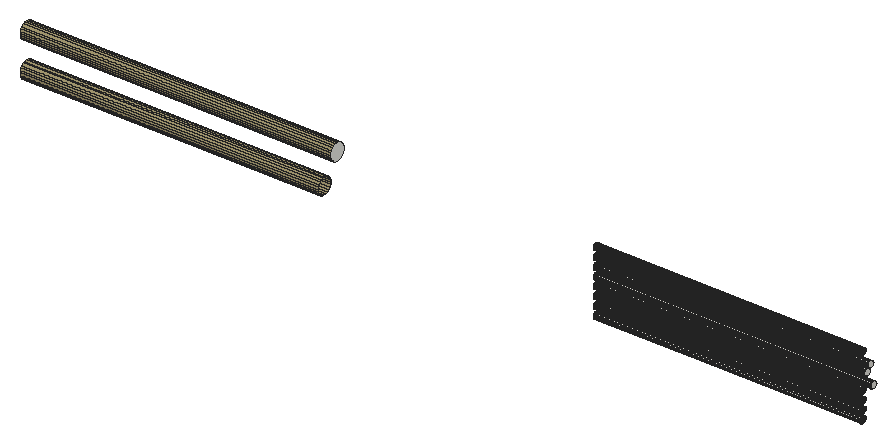
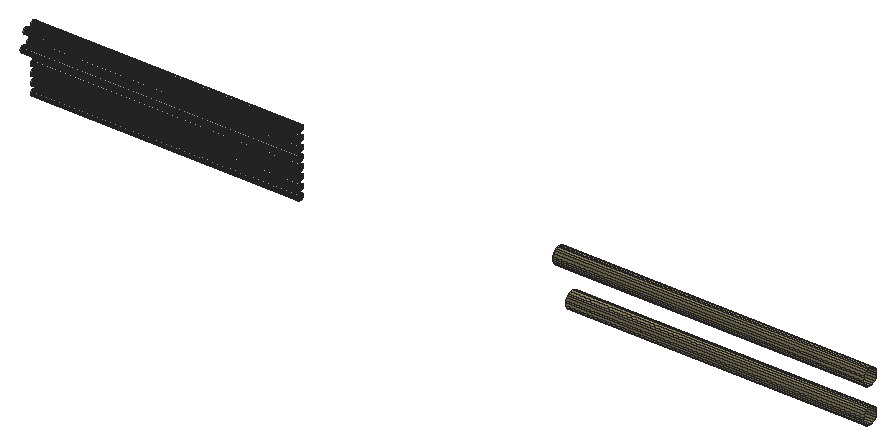
# SketchUp Ruby script. Lengths in inches.
U = 1.inch
M = Sketchup.active_model
def pt(a) = Geom::Point3d.new(a.map { |v| v * U })
def face(e, loops, mat)
  f = e.add_face(loops[0].map { |a| pt(a) })
  loops[1..].each { |l| e.add_face(l.map { |a| pt(a) }).erase! }
  f.material = f.back_material = mat if mat
  f
end
# faces: each face lists its corners as indices into pts; further lists are holes
def faces(e, pts, list, mat = nil) = list.each { |f| face(e, (f[0].is_a?(Array) ? f : [f]).map { |l| l.map { |i| pts[i] } }, mat) }
# xy, xz, yz: faces in a plane at the given z, y or x. An outline is a flat list of corners, or four numbers for a rectangle; further outlines are holes
def ring(l) = l.size == 4 ? [[l[0], l[1]], [l[2], l[1]], [l[2], l[3]], [l[0], l[3]]] : l.each_slice(2).to_a
def flat(e, list, mat, &to3) = list.each { |f| face(e, (f[0].is_a?(Array) ? f : [f]).map { |l| ring(l).map { |u, v| to3.(u, v) } }, mat) }
def xy(e, z, list, mat = nil) = flat(e, list, mat) { |x, y| [x, y, z] }
def xz(e, y, list, mat = nil) = flat(e, list, mat) { |x, z| [x, y, z] }
def yz(e, x, list, mat = nil) = flat(e, list, mat) { |y, z| [x, y, z] }
def lines(e, pts, list) = list.each { |a, b| e.add_line(pt(pts[a]), pt(pts[b])) }
# prism: a flat outline (further loops are holes) pulled along v
def prism(e, loops, v, mat = nil)
  f = face(e, loops, mat); d = Geom::Vector3d.new(v.map { |x| x * U })
  f.pushpull(f.normal.samedirection?(d) ? d.length : -d.length)
end
def box(e, o, s, mat = nil) = prism(e, [[o, [o[0] + s[0], o[1], o[2]], [o[0] + s[0], o[1] + s[1], o[2]], [o[0], o[1] + s[1], o[2]]]], [0, 0, s[2]], mat)
def at(x, y, z, deg = 0) = Geom::Transformation.translation(pt([x, y, z])) * Geom::Transformation.rotation(ORIGIN, Z_AXIS, deg.degrees)
def axes(o, x, y, z) = Geom::Transformation.new([*x, 0, *y, 0, *z, 0, *pt(o).to_a, 1])
def part(name) = M.definitions.add(name)
# library, detail: a bought-in or finely detailed component or shape, given as its bounding box
def library(name, o, s) = part(name).tap { |d| box(d.entities, o, s) }
def detail(e, o, s) = box(e.add_group.entities, o, s)
def put(e, d, t, mat = nil) = e.add_instance(d, t).tap { |i| i.material = mat if mat }
def group(e, t, mat = nil) = e.add_group.tap { |g| g.transformation = t; g.material = mat if mat }.entities
root = M.entities
M.materials.add("[Terrazzo Tile Light]").color = [219, 217, 210]
M.materials.add("[Wood Lumber ButtJoined]").color = [164, 152, 112]
yz(root,389.28,[[249.32,189.85,249.99,189.94,250.6,190.2,251.14,190.6,251.54,191.13,251.8,191.75,251.89,192.42,251.8,193.08,251.54,193.7,251.14,194.23,250.6,194.63,249.99,194.89,249.32,194.98,248.66,194.89,248.04,194.63,247.51,194.23,247.1,193.7,246.85,193.08,246.76,192.42,246.85,191.75,247.1,191.13,247.51,190.6,248.04,190.2,248.66,189.94]])
yz(root,558.48,[[245.69,190.45,245.94,190.48,246.16,190.58,246.36,190.73,246.5,190.92,246.6,191.15,246.63,191.39,246.6,191.63,246.5,191.86,246.36,192.05,246.16,192.2,245.94,192.29,245.69,192.33,245.45,192.29,245.22,192.2,245.03,192.05,244.88,191.86,244.79,191.63,244.75,191.39,244.79,191.15,244.88,190.92,245.03,190.73,245.22,190.58,245.45,190.48]],"[Terrazzo Tile Light]")
yz(root,559.54,[[245.69,193.2,245.94,193.23,246.16,193.33,246.36,193.48,246.5,193.67,246.6,193.9,246.63,194.14,246.6,194.38,246.5,194.61,246.36,194.8,246.16,194.95,245.94,195.04,245.69,195.08,245.45,195.04,245.22,194.95,245.03,194.8,244.88,194.61,244.79,194.38,244.75,194.14,244.79,193.9,244.88,193.67,245.03,193.48,245.22,193.33,245.45,193.23]],"[Terrazzo Tile Light]")
yz(root,560.48,[[245.69,187.7,245.94,187.73,246.16,187.83,246.36,187.98,246.5,188.17,246.6,188.4,246.63,188.64,246.6,188.88,246.5,189.11,246.36,189.3,246.16,189.45,245.94,189.54,245.69,189.58,245.45,189.54,245.22,189.45,245.03,189.3,244.88,189.11,244.79,188.88,244.75,188.64,244.79,188.4,244.88,188.17,245.03,187.98,245.22,187.83,245.45,187.73]],"[Terrazzo Tile Light]")
p = [[473.23,245.22,176.83],[473.23,245.45,176.73],[557.23,245.45,176.73],[557.23,245.22,176.83],[473.23,245.69,176.7],[557.23,245.69,176.7],
  [473.23,245.94,176.73],[557.23,245.94,176.73],[473.23,246.16,176.83],[557.23,246.16,176.83],[473.23,245.03,176.98],[557.23,245.03,176.98],
  [473.23,246.36,176.98],[557.23,246.36,176.98],[473.23,244.88,177.17],[557.23,244.88,177.17],[473.23,246.5,177.17],[557.23,246.5,177.17],
  [473.23,244.79,177.4],[557.23,244.79,177.4],[473.23,246.6,177.4],[557.23,246.6,177.4],[473.23,244.75,177.64],[557.23,244.75,177.64],
  [473.23,246.63,177.64],[557.23,246.63,177.64],[473.23,244.79,177.88],[557.23,244.79,177.88],[473.23,246.6,177.88],[557.23,246.6,177.88],
  [473.23,244.88,178.11],[557.23,244.88,178.11],[473.23,246.5,178.11],[557.23,246.5,178.11],[473.23,245.03,178.3],[557.23,245.03,178.3],
  [473.23,246.36,178.3],[557.23,246.36,178.3],[473.23,245.22,178.45],[557.23,245.22,178.45],[473.23,246.16,178.45],[557.23,246.16,178.45],
  [473.23,245.45,178.54],[557.23,245.45,178.54],[473.23,245.69,178.58],[557.23,245.69,178.58],[473.23,245.94,178.54],[557.23,245.94,178.54],
  [291.78,248.04,179.2],[291.78,248.66,178.94],[385.09,248.66,178.94],[385.09,248.04,179.2],[291.78,249.32,178.85],[385.09,249.32,178.85],
  [291.78,249.99,178.94],[385.09,249.99,178.94],[291.78,250.6,179.2],[385.09,250.6,179.2],[291.78,247.51,179.6],[385.09,247.51,179.6],
  [291.78,251.14,179.6],[385.09,251.14,179.6],[473.23,245.22,179.58],[473.23,245.45,179.48],[557.23,245.45,179.48],[557.23,245.22,179.58],
  [473.23,245.69,179.45],[557.23,245.69,179.45],[473.23,245.94,179.48],[557.23,245.94,179.48],[473.23,246.16,179.58],[557.23,246.16,179.58],
  [473.23,245.03,179.73],[557.23,245.03,179.73],[473.23,246.36,179.73],[557.23,246.36,179.73],[291.78,247.1,180.13],[385.09,247.1,180.13],
  [291.78,251.54,180.13],[385.09,251.54,180.13],[473.23,244.88,179.92],[557.23,244.88,179.92],[473.23,246.5,179.92],[557.23,246.5,179.92],
  [473.23,244.79,180.15],[557.23,244.79,180.15],[473.23,246.6,180.15],[557.23,246.6,180.15],[473.23,244.75,180.39],[557.23,244.75,180.39],
  [473.23,246.63,180.39],[557.23,246.63,180.39],[291.78,246.85,180.75],[385.09,246.85,180.75],[291.78,251.8,180.75],[385.09,251.8,180.75],
  [473.23,244.79,180.63],[557.23,244.79,180.63],[473.23,246.6,180.63],[557.23,246.6,180.63],[473.23,244.88,180.86],[557.23,244.88,180.86],
  [473.23,246.5,180.86],[557.23,246.5,180.86],[291.78,246.76,181.42],[385.09,246.76,181.42],[291.78,251.89,181.42],[385.09,251.89,181.42],
  [473.23,245.03,181.05],[557.23,245.03,181.05],[473.23,246.36,181.05],[557.23,246.36,181.05],[473.23,245.22,181.2],[557.23,245.22,181.2],
  [473.23,246.16,181.2],[557.23,246.16,181.2],[473.23,245.45,181.29],[557.23,245.45,181.29],[473.23,245.94,181.29],[557.23,245.94,181.29],
  [473.23,245.69,181.33],[557.23,245.69,181.33],[291.78,246.85,182.08],[385.09,246.85,182.08],[291.78,251.8,182.08],[385.09,251.8,182.08],
  [291.78,247.1,182.7],[385.09,247.1,182.7],[291.78,251.54,182.7],[385.09,251.54,182.7],[473.23,245.22,182.33],[473.23,245.45,182.23],
  [557.23,245.45,182.23],[557.23,245.22,182.33],[473.23,245.69,182.2],[557.23,245.69,182.2],[473.23,245.94,182.23],[557.23,245.94,182.23],
  [473.23,246.16,182.33],[557.23,246.16,182.33],[473.23,245.03,182.48],[557.23,245.03,182.48],[473.23,246.36,182.48],[557.23,246.36,182.48],
  [473.23,244.88,182.67],[557.23,244.88,182.67],[473.23,246.5,182.67],[557.23,246.5,182.67],[473.23,244.79,182.9],[557.23,244.79,182.9],
  [473.23,246.6,182.9],[557.23,246.6,182.9],[291.78,247.51,183.23],[385.09,247.51,183.23],[291.78,251.14,183.23],[385.09,251.14,183.23],
  [473.23,244.75,183.14],[557.23,244.75,183.14],[473.23,246.63,183.14],[557.23,246.63,183.14],[473.23,244.79,183.38],[557.23,244.79,183.38],
  [473.23,246.6,183.38],[557.23,246.6,183.38],[291.78,248.04,183.63],[385.09,248.04,183.63],[291.78,250.6,183.63],[385.09,250.6,183.63],
  [473.23,244.88,183.61],[557.23,244.88,183.61],[473.23,246.5,183.61],[557.23,246.5,183.61],[473.23,245.03,183.8],[557.23,245.03,183.8],
  [473.23,246.36,183.8],[557.23,246.36,183.8],[291.78,248.66,183.89],[385.09,248.66,183.89],[291.78,249.99,183.89],[385.09,249.99,183.89],
  [473.23,245.22,183.95],[557.23,245.22,183.95],[473.23,246.16,183.95],[557.23,246.16,183.95],[291.78,249.32,183.98],[385.09,249.32,183.98],
  [473.23,245.45,184.04],[557.23,245.45,184.04],[473.23,245.69,184.08],[557.23,245.69,184.08],[473.23,245.94,184.04],[557.23,245.94,184.04],
  [473.23,245.22,185.08],[473.23,245.45,184.98],[557.23,245.45,184.98],[557.23,245.22,185.08],[473.23,245.69,184.95],[557.23,245.69,184.95],
  [473.23,245.94,184.98],[557.23,245.94,184.98],[473.23,246.16,185.08],[557.23,246.16,185.08],[473.23,245.03,185.23],[557.23,245.03,185.23],
  [473.23,246.36,185.23],[557.23,246.36,185.23],[473.23,244.88,185.42],[557.23,244.88,185.42],[473.23,246.5,185.42],[557.23,246.5,185.42],
  [473.23,244.79,185.65],[557.23,244.79,185.65],[473.23,246.6,185.65],[557.23,246.6,185.65],[473.23,244.75,185.89],[557.23,244.75,185.89],
  [473.23,246.63,185.89],[557.23,246.63,185.89],[473.23,244.79,186.13],[557.23,244.79,186.13],[473.23,246.6,186.13],[557.23,246.6,186.13],
  [473.23,244.88,186.36],[557.23,244.88,186.36],[473.23,246.5,186.36],[557.23,246.5,186.36],[473.23,245.03,186.55],[557.23,245.03,186.55],
  [473.23,246.36,186.55],[557.23,246.36,186.55],[473.23,245.22,186.7],[557.23,245.22,186.7],[473.23,246.16,186.7],[557.23,246.16,186.7],
  [473.23,245.45,186.79],[557.23,245.45,186.79],[473.23,245.94,186.79],[557.23,245.94,186.79],[473.23,245.69,186.83],[557.23,245.69,186.83],
  [473.23,245.22,187.83],[473.23,245.45,187.73],[560.48,245.45,187.73],[560.48,245.22,187.83],[473.23,245.69,187.7],[560.48,245.69,187.7],
  [473.23,245.94,187.73],[560.48,245.94,187.73],[473.23,246.16,187.83],[560.48,246.16,187.83],[473.23,245.03,187.98],[560.48,245.03,187.98],
  [473.23,246.36,187.98],[560.48,246.36,187.98],[473.23,244.88,188.17],[560.48,244.88,188.17],[473.23,246.5,188.17],[560.48,246.5,188.17],
  [473.23,244.79,188.4],[560.48,244.79,188.4],[473.23,246.6,188.4],[560.48,246.6,188.4],[473.23,244.75,188.64],[560.48,244.75,188.64],
  [473.23,246.63,188.64],[560.48,246.63,188.64],[473.23,244.79,188.88],[560.48,244.79,188.88],[473.23,246.6,188.88],[560.48,246.6,188.88],
  [473.23,244.88,189.11],[560.48,244.88,189.11],[473.23,246.5,189.11],[560.48,246.5,189.11],[473.23,245.03,189.3],[560.48,245.03,189.3],
  [473.23,246.36,189.3],[560.48,246.36,189.3],[473.23,245.22,189.45],[560.48,245.22,189.45],[473.23,246.16,189.45],[560.48,246.16,189.45],
  [473.23,245.45,189.54],[560.48,245.45,189.54],[473.23,245.69,189.58],[560.48,245.69,189.58],[473.23,245.94,189.54],[560.48,245.94,189.54],
  [291.78,248.04,190.2],[291.78,248.66,189.94],[389.28,248.66,189.94],[389.28,248.04,190.2],[291.78,249.32,189.85],[389.28,249.32,189.85],
  [291.78,249.99,189.94],[389.28,249.99,189.94],[291.78,250.6,190.2],[389.28,250.6,190.2],[291.78,247.51,190.6],[389.28,247.51,190.6],
  [291.78,251.14,190.6],[389.28,251.14,190.6],[473.23,245.22,190.58],[473.23,245.45,190.48],[558.48,245.45,190.48],[558.48,245.22,190.58],
  [473.23,245.69,190.45],[558.48,245.69,190.45],[473.23,245.94,190.48],[558.48,245.94,190.48],[473.23,246.16,190.58],[558.48,246.16,190.58],
  [473.23,245.03,190.73],[558.48,245.03,190.73],[473.23,246.36,190.73],[558.48,246.36,190.73],[291.78,247.1,191.13],[389.28,247.1,191.13],
  [291.78,251.54,191.13],[389.28,251.54,191.13],[473.23,244.88,190.92],[558.48,244.88,190.92],[473.23,246.5,190.92],[558.48,246.5,190.92],
  [473.23,244.79,191.15],[558.48,244.79,191.15],[473.23,246.6,191.15],[558.48,246.6,191.15],[473.23,244.75,191.39],[558.48,244.75,191.39],
  [473.23,246.63,191.39],[558.48,246.63,191.39],[291.78,246.85,191.75],[389.28,246.85,191.75],[291.78,251.8,191.75],[389.28,251.8,191.75],
  [473.23,244.79,191.63],[558.48,244.79,191.63],[473.23,246.6,191.63],[558.48,246.6,191.63],[473.23,244.88,191.86],[558.48,244.88,191.86],
  [473.23,246.5,191.86],[558.48,246.5,191.86],[291.78,246.76,192.42],[389.28,246.76,192.42],[291.78,251.89,192.42],[389.28,251.89,192.42],
  [473.23,245.03,192.05],[558.48,245.03,192.05],[473.23,246.36,192.05],[558.48,246.36,192.05],[473.23,245.22,192.2],[558.48,245.22,192.2],
  [473.23,246.16,192.2],[558.48,246.16,192.2],[473.23,245.45,192.29],[558.48,245.45,192.29],[473.23,245.94,192.29],[558.48,245.94,192.29],
  [473.23,245.69,192.33],[558.48,245.69,192.33],[291.78,246.85,193.08],[389.28,246.85,193.08],[291.78,251.8,193.08],[389.28,251.8,193.08],
  [291.78,247.1,193.7],[389.28,247.1,193.7],[291.78,251.54,193.7],[389.28,251.54,193.7],[473.23,245.22,193.33],[473.23,245.45,193.23],
  [559.54,245.45,193.23],[559.54,245.22,193.33],[473.23,245.69,193.2],[559.54,245.69,193.2],[473.23,245.94,193.23],[559.54,245.94,193.23],
  [473.23,246.16,193.33],[559.54,246.16,193.33],[473.23,245.03,193.48],[559.54,245.03,193.48],[473.23,246.36,193.48],[559.54,246.36,193.48],
  [473.23,244.88,193.67],[559.54,244.88,193.67],[473.23,246.5,193.67],[559.54,246.5,193.67],[473.23,244.79,193.9],[559.54,244.79,193.9],
  [473.23,246.6,193.9],[559.54,246.6,193.9],[291.78,247.51,194.23],[389.28,247.51,194.23],[291.78,251.14,194.23],[389.28,251.14,194.23],
  [473.23,244.75,194.14],[559.54,244.75,194.14],[473.23,246.63,194.14],[559.54,246.63,194.14],[473.23,244.79,194.38],[559.54,244.79,194.38],
  [473.23,246.6,194.38],[559.54,246.6,194.38],[291.78,248.04,194.63],[389.28,248.04,194.63],[291.78,250.6,194.63],[389.28,250.6,194.63],
  [473.23,244.88,194.61],[559.54,244.88,194.61],[473.23,246.5,194.61],[559.54,246.5,194.61],[473.23,245.03,194.8],[559.54,245.03,194.8],
  [473.23,246.36,194.8],[559.54,246.36,194.8],[291.78,248.66,194.89],[389.28,248.66,194.89],[291.78,249.99,194.89],[389.28,249.99,194.89],
  [473.23,245.22,194.95],[559.54,245.22,194.95],[473.23,246.16,194.95],[559.54,246.16,194.95],[291.78,249.32,194.98],[389.28,249.32,194.98],
  [473.23,245.45,195.04],[559.54,245.45,195.04],[473.23,245.69,195.08],[559.54,245.69,195.08],[473.23,245.94,195.04],[559.54,245.94,195.04],
  [473.23,245.22,196.08],[473.23,245.45,195.98],[557.23,245.45,195.98],[557.23,245.22,196.08],[473.23,245.69,195.95],[557.23,245.69,195.95],
  [473.23,245.94,195.98],[557.23,245.94,195.98],[473.23,246.16,196.08],[557.23,246.16,196.08],[473.23,245.03,196.23],[557.23,245.03,196.23],
  [473.23,246.36,196.23],[557.23,246.36,196.23],[473.23,244.88,196.42],[557.23,244.88,196.42],[473.23,246.5,196.42],[557.23,246.5,196.42],
  [473.23,244.79,196.65],[557.23,244.79,196.65],[473.23,246.6,196.65],[557.23,246.6,196.65],[473.23,244.75,196.89],[557.23,244.75,196.89],
  [473.23,246.63,196.89],[557.23,246.63,196.89],[473.23,244.79,197.13],[557.23,244.79,197.13],[473.23,246.6,197.13],[557.23,246.6,197.13],
  [473.23,244.88,197.36],[557.23,244.88,197.36],[473.23,246.5,197.36],[557.23,246.5,197.36],[473.23,245.03,197.55],[557.23,245.03,197.55],
  [473.23,246.36,197.55],[557.23,246.36,197.55],[473.23,245.22,197.7],[557.23,245.22,197.7],[473.23,246.16,197.7],[557.23,246.16,197.7],
  [473.23,245.45,197.79],[557.23,245.45,197.79],[473.23,245.94,197.79],[557.23,245.94,197.79],[473.23,245.69,197.83],[557.23,245.69,197.83]]
faces(root,p,[[0,1,2,3],[1,4,5,2],[4,6,7,5],[6,8,9,7],[10,0,3,11],[8,12,13,9],[14,10,11,15],[12,16,17,13],
  [18,14,15,19],[16,20,21,17],[22,18,19,23],[20,24,25,21],[26,22,23,27],[24,28,29,25],[30,26,27,31],[28,32,33,29],
  [34,30,31,35],[32,36,37,33],[38,34,35,39],[36,40,41,37],[42,38,39,43],[44,42,43,45],[46,44,45,47],[40,46,47,41],
  [62,63,64,65],[63,66,67,64],[66,68,69,67],[68,70,71,69],[72,62,65,73],[70,74,75,71],[80,72,73,81],[74,82,83,75],
  [84,80,81,85],[82,86,87,83],[88,84,85,89],[86,90,91,87],[96,88,89,97],[90,98,99,91],[100,96,97,101],[98,102,103,99],
  [108,100,101,109],[102,110,111,103],[112,108,109,113],[110,114,115,111],[116,112,113,117],[114,118,119,115],[120,116,117,121],[118,120,121,119],
  [130,131,132,133],[131,134,135,132],[134,136,137,135],[136,138,139,137],[140,130,133,141],[138,142,143,139],[144,140,141,145],[142,146,147,143],
  [148,144,145,149],[146,150,151,147],[156,148,149,157],[150,158,159,151],[160,156,157,161],[158,162,163,159],[168,160,161,169],[162,170,171,163],
  [172,168,169,173],[170,174,175,171],[180,172,173,181],[174,182,183,175],[186,180,181,187],[188,186,187,189],[190,188,189,191],[182,190,191,183],
  [192,193,194,195],[193,196,197,194],[196,198,199,197],[198,200,201,199],[202,192,195,203],[200,204,205,201],[206,202,203,207],[204,208,209,205],
  [210,206,207,211],[208,212,213,209],[214,210,211,215],[212,216,217,213],[218,214,215,219],[216,220,221,217],[222,218,219,223],[220,224,225,221],
  [226,222,223,227],[224,228,229,225],[230,226,227,231],[228,232,233,229],[234,230,231,235],[232,236,237,233],[238,234,235,239],[236,238,239,237],
  [240,241,242,243],[241,244,245,242],[244,246,247,245],[246,248,249,247],[250,240,243,251],[248,252,253,249],[254,250,251,255],[252,256,257,253],
  [258,254,255,259],[256,260,261,257],[262,258,259,263],[260,264,265,261],[266,262,263,267],[264,268,269,265],[270,266,267,271],[268,272,273,269],
  [274,270,271,275],[272,276,277,273],[278,274,275,279],[276,280,281,277],[282,278,279,283],[284,282,283,285],[286,284,285,287],[280,286,287,281],
  [302,303,304,305],[303,306,307,304],[306,308,309,307],[308,310,311,309],[312,302,305,313],[310,314,315,311],[320,312,313,321],[314,322,323,315],
  [324,320,321,325],[322,326,327,323],[328,324,325,329],[326,330,331,327],[336,328,329,337],[330,338,339,331],[340,336,337,341],[338,342,343,339],
  [348,340,341,349],[342,350,351,343],[352,348,349,353],[350,354,355,351],[356,352,353,357],[354,358,359,355],[360,356,357,361],[358,360,361,359],
  [370,371,372,373],[371,374,375,372],[374,376,377,375],[376,378,379,377],[380,370,373,381],[378,382,383,379],[384,380,381,385],[382,386,387,383],
  [388,384,385,389],[386,390,391,387],[396,388,389,397],[390,398,399,391],[400,396,397,401],[398,402,403,399],[408,400,401,409],[402,410,411,403],
  [412,408,409,413],[410,414,415,411],[420,412,413,421],[414,422,423,415],[426,420,421,427],[428,426,427,429],[430,428,429,431],[422,430,431,423],
  [432,433,434,435],[433,436,437,434],[436,438,439,437],[438,440,441,439],[442,432,435,443],[440,444,445,441],[446,442,443,447],[444,448,449,445],
  [450,446,447,451],[448,452,453,449],[454,450,451,455],[452,456,457,453],[458,454,455,459],[456,460,461,457],[462,458,459,463],[460,464,465,461],
  [466,462,463,467],[464,468,469,465],[470,466,467,471],[468,472,473,469],[474,470,471,475],[472,476,477,473],[478,474,475,479],[476,478,479,477]],"[Terrazzo Tile Light]")
faces(root,p,[[48,49,50,51],[49,52,53,50],[52,54,55,53],[54,56,57,55],[58,48,51,59],[56,60,61,57],[76,58,59,77],[60,78,79,61],
  [92,76,77,93],[78,94,95,79],[104,92,93,105],[94,106,107,95],[122,104,105,123],[106,124,125,107],[126,122,123,127],[124,128,129,125],
  [152,126,127,153],[128,154,155,129],[164,152,153,165],[154,166,167,155],[176,164,165,177],[166,178,179,167],[184,176,177,185],[178,184,185,179],
  [288,289,290,291],[289,292,293,290],[292,294,295,293],[294,296,297,295],[298,288,291,299],[296,300,301,297],[316,298,299,317],[300,318,319,301],
  [332,316,317,333],[318,334,335,319],[344,332,333,345],[334,346,347,335],[362,344,345,363],[346,364,365,347],[366,362,363,367],[364,368,369,365],
  [392,366,367,393],[368,394,395,369],[404,392,393,405],[394,406,407,395],[416,404,405,417],[406,418,419,407],[424,416,417,425],[418,424,425,419]],"[Wood Lumber ButtJoined]")
